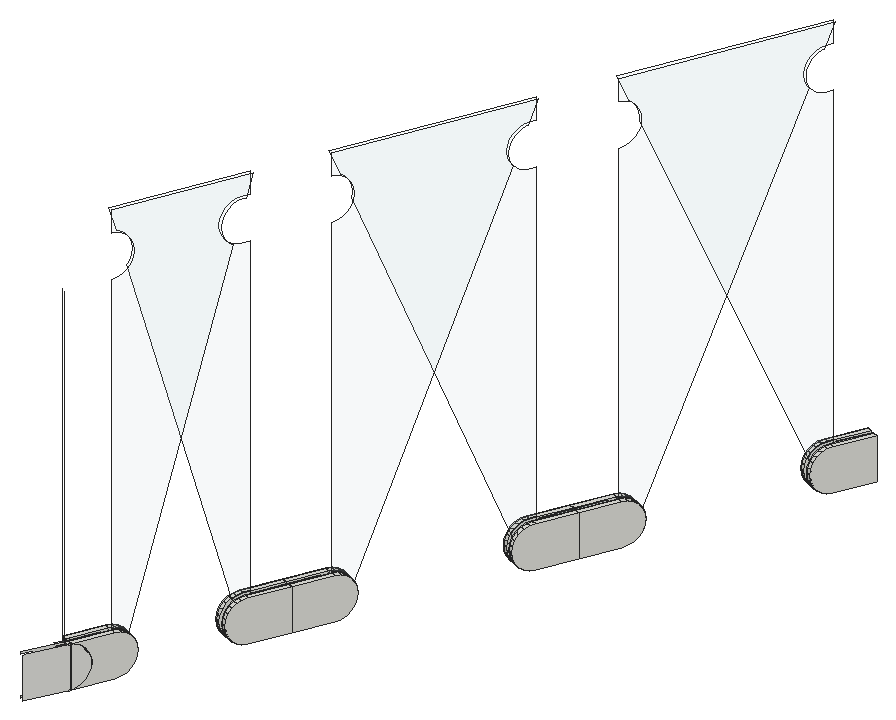
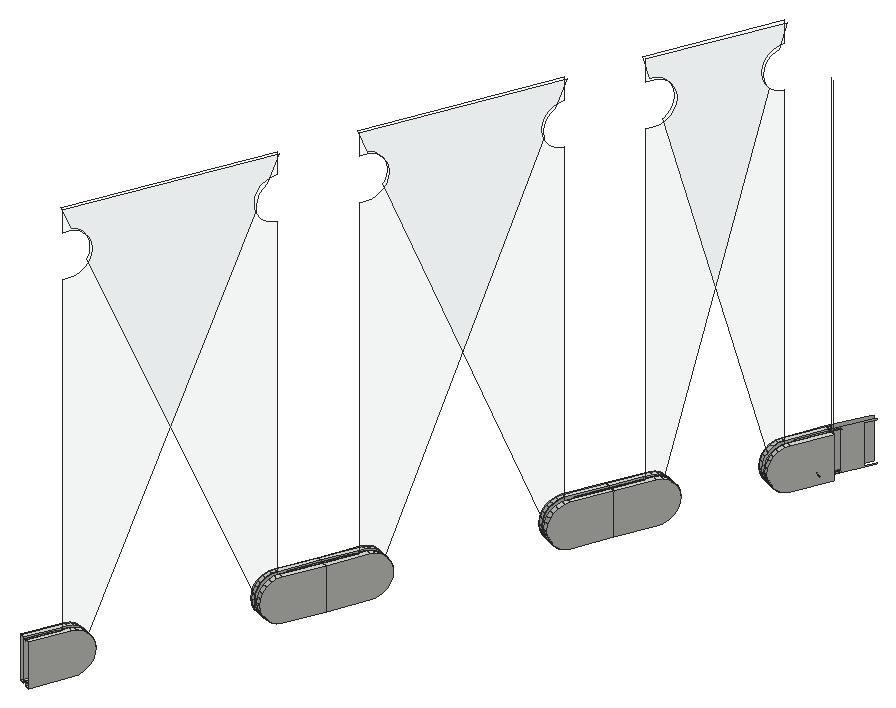
# SketchUp Ruby script. Lengths in inches.
U = 1.inch
M = Sketchup.active_model
def pt(a) = Geom::Point3d.new(a.map { |v| v * U })
def face(e, loops, mat)
  f = e.add_face(loops[0].map { |a| pt(a) })
  loops[1..].each { |l| e.add_face(l.map { |a| pt(a) }).erase! }
  f.material = f.back_material = mat if mat
  f
end
# faces: each face lists its corners as indices into pts; further lists are holes
def faces(e, pts, list, mat = nil) = list.each { |f| face(e, (f[0].is_a?(Array) ? f : [f]).map { |l| l.map { |i| pts[i] } }, mat) }
# xy, xz, yz: faces in a plane at the given z, y or x. An outline is a flat list of corners, or four numbers for a rectangle; further outlines are holes
def ring(l) = l.size == 4 ? [[l[0], l[1]], [l[2], l[1]], [l[2], l[3]], [l[0], l[3]]] : l.each_slice(2).to_a
def flat(e, list, mat, &to3) = list.each { |f| face(e, (f[0].is_a?(Array) ? f : [f]).map { |l| ring(l).map { |u, v| to3.(u, v) } }, mat) }
def xy(e, z, list, mat = nil) = flat(e, list, mat) { |x, y| [x, y, z] }
def xz(e, y, list, mat = nil) = flat(e, list, mat) { |x, z| [x, y, z] }
def yz(e, x, list, mat = nil) = flat(e, list, mat) { |y, z| [x, y, z] }
def lines(e, pts, list) = list.each { |a, b| e.add_line(pt(pts[a]), pt(pts[b])) }
# prism: a flat outline (further loops are holes) pulled along v
def prism(e, loops, v, mat = nil)
  f = face(e, loops, mat); d = Geom::Vector3d.new(v.map { |x| x * U })
  f.pushpull(f.normal.samedirection?(d) ? d.length : -d.length)
end
def box(e, o, s, mat = nil) = prism(e, [[o, [o[0] + s[0], o[1], o[2]], [o[0] + s[0], o[1] + s[1], o[2]], [o[0], o[1] + s[1], o[2]]]], [0, 0, s[2]], mat)
def at(x, y, z, deg = 0) = Geom::Transformation.translation(pt([x, y, z])) * Geom::Transformation.rotation(ORIGIN, Z_AXIS, deg.degrees)
def axes(o, x, y, z) = Geom::Transformation.new([*x, 0, *y, 0, *z, 0, *pt(o).to_a, 1])
def part(name) = M.definitions.add(name)
# library, detail: a bought-in or finely detailed component or shape, given as its bounding box
def library(name, o, s) = part(name).tap { |d| box(d.entities, o, s) }
def detail(e, o, s) = box(e.add_group.entities, o, s)
def put(e, d, t, mat = nil) = e.add_instance(d, t).tap { |i| i.material = mat if mat }
def group(e, t, mat = nil) = e.add_group.tap { |g| g.transformation = t; g.material = mat if mat }.entities
root = M.entities
M.materials.add("Glass_Safety_01").color = [204, 235, 244]
M.materials["Glass_Safety_01"].alpha = 0.1
xy(root,333,[[844.286,537.43,844.039,537.551,844.044,537.562,844.108,537.692,844.355,537.571],[844.362,537.586,844.11,537.696,844.896,539.501,845.148,539.391],[843.931,537.779,843.684,537.9,844.463,539.689,844.715,539.579],[847.571,544.953,847.318,545.063,847.473,545.418,848.104,546.868,848.357,546.758],[847.138,545.142,846.885,545.252,847.671,547.057,847.924,546.947,847.293,545.497,847.167,545.208],
  [848.357,546.758,848.104,546.868,848.89,548.673,849.143,548.563],[847.924,546.947,847.671,547.057,848.457,548.861,848.71,548.751],[852.79,556.936,852.537,557.046,852.656,557.318,853.323,558.851,853.576,558.741],[852.357,557.125,852.104,557.235,852.89,559.04,853.143,558.93,852.475,557.397],[853.576,558.741,853.323,558.851,854.109,560.656,854.362,560.546],
  [853.143,558.93,852.89,559.04,853.676,560.845,853.929,560.735],[858.192,569.34,857.939,569.45,858.054,569.713,858.726,571.255,858.978,571.145],[857.759,569.529,857.506,569.639,858.292,571.443,858.545,571.333,857.873,569.791]])
xy(root,333.078,[[843.866,537.198,843.689,537.285,843.862,537.638,843.867,537.648,843.929,537.775,844.019,537.735,844.108,537.692,844.044,537.562,844.039,537.552],[844.11,537.696,844.019,537.735,843.931,537.779,844.558,539.218,844.738,539.14],[844.019,537.735,843.929,537.775,843.931,537.779],[847.476,545.424,847.295,545.503,847.924,546.947,848.104,546.868],[848.104,546.868,847.924,546.947,848.553,548.39,848.733,548.312],
  [852.695,557.407,852.514,557.486,853.143,558.93,853.323,558.851],[853.323,558.851,853.143,558.93,853.772,560.374,853.952,560.295],[858.097,569.811,857.916,569.89,858.545,571.333,858.726,571.255]],"Glass_Safety_01")
xy(root,335.047,[[843.866,537.198,844.039,537.551,844.04,537.553,844.044,537.562,844.108,537.692,844.019,537.735,843.929,537.775,843.867,537.648,843.867,537.647,843.862,537.638,843.689,537.285],[844.11,537.696,844.738,539.14,844.558,539.218,843.931,537.779,844.019,537.735],[844.019,537.735,843.931,537.779,843.929,537.775],[847.476,545.424,848.104,546.868,847.924,546.947,847.295,545.503],[848.104,546.868,848.733,548.312,848.553,548.39,847.924,546.947],
  [852.695,557.407,853.323,558.851,853.143,558.93,852.514,557.486],[853.323,558.851,853.952,560.295,853.772,560.374,853.143,558.93],[858.097,569.811,858.726,571.255,858.545,571.333,857.916,569.89]],"Glass_Safety_01")
xy(root,335.126,[[844.362,537.586,845.148,539.391,844.896,539.501,844.11,537.696],[843.931,537.779,844.715,539.579,844.463,539.689,843.684,537.9],[847.571,544.953,848.357,546.758,848.104,546.868,847.473,545.418,847.318,545.063],[847.138,545.142,847.293,545.497,847.924,546.947,847.671,547.057,846.885,545.252],[848.357,546.758,849.143,548.563,848.89,548.673,848.104,546.868],
  [847.924,546.947,848.71,548.751,848.457,548.861,847.671,547.057],[852.79,556.936,853.576,558.741,853.323,558.851,852.656,557.318,852.537,557.046],[852.357,557.125,852.475,557.397,853.143,558.93,852.89,559.04,852.104,557.235],[853.576,558.741,854.362,560.546,854.109,560.656,853.323,558.851],[853.143,558.93,853.929,560.735,853.676,560.845,852.89,559.04],
  [858.192,569.34,858.978,571.145,858.726,571.255,858.054,569.713,857.939,569.45],[857.759,569.529,857.873,569.791,858.545,571.333,858.292,571.443,857.506,569.639]])
yz(root,843.867,[[537.648,333.078,537.647,335.047,537.648,335.047]],"Glass_Safety_01")
p = [[843.42,535.662,335.105],[843.42,535.662,333.02],[843.489,535.803,333],[844.286,537.43,333],[844.355,537.571,333.02],[844.355,537.571,335.105],
  [844.286,537.43,335.126],[843.489,535.803,335.126],[843.173,535.784,335.047],[843.173,535.784,335.105],[843.242,535.924,335.126],[844.039,537.551,335.126],
  [844.04,537.553,335.125],[844.044,537.562,335.124],[844.108,537.692,335.105],[844.108,537.692,335.047],[844.044,537.562,335.047],[844.044,537.562,333.078],
  [844.108,537.692,333.078],[844.11,537.696,335.104],[844.16,537.799,335.089],[844.273,538.029,334.983],[844.37,538.226,334.814],[844.444,538.378,334.594],
  [844.491,538.474,334.338],[844.507,538.506,334.0625],[844.491,538.474,333.787],[844.444,538.378,333.531],[844.37,538.226,333.311],[844.273,538.029,333.142],
  [844.16,537.799,333.036],[844.11,537.696,333.021],[844.108,537.692,333.02],[844.044,537.562,333.001],[844.039,537.551,333],[843.242,535.924,333],
  [843.173,535.784,333.02],[843.173,535.784,333.078],[843.415,536.278,333.078],[843.415,536.278,335.047],[844.04,537.553,335.047],[844.039,537.551,335.047],
  [843.866,537.198,335.047],[843.866,537.198,333.078],[844.039,537.552,333.078],[844.407,537.677,333.036],[844.362,537.586,333.022],[844.355,537.571,333],
  [843.867,537.648,333.001],[843.867,537.648,333],[843.862,537.638,333],[843.862,537.638,333.078],[843.867,537.648,333.078],[844.044,537.562,333],
  [844.108,537.692,333],[844.108,537.692,335.126],[844.355,537.571,335.126],[844.11,537.696,333],[844.362,537.586,333],[844.362,537.586,335.103],
  [844.362,537.586,335.126],[844.11,537.696,335.126],[844.11,537.696,335.047],[844.11,537.696,333.078],[844.407,537.677,335.089],[844.52,537.908,333.142],
  [844.617,538.105,333.311],[844.691,538.257,333.531],[844.738,538.352,333.787],[844.754,538.385,334.0625],[844.738,538.352,334.338],[844.691,538.257,334.594],
  [844.617,538.105,334.814],[844.52,537.908,334.983],[845.148,539.391,335.126],[845.148,539.391,333],[845.258,539.643,333.036],[845.361,539.878,333.142],
  [845.448,540.08,333.311],[845.516,540.235,333.531],[845.558,540.332,333.787],[845.573,540.365,334.0625],[845.558,540.332,334.338],[845.516,540.235,334.594],
  [845.448,540.08,334.814],[845.361,539.878,334.983],[845.258,539.643,335.089],[844.896,539.501,335.126],[845.006,539.753,335.089],[845.108,539.988,334.983],
  [845.196,540.19,334.814],[845.219,540.244,334.737],[845.263,540.345,334.594],[845.306,540.442,334.338],[845.32,540.475,334.0625],[845.306,540.442,333.787],
  [845.263,540.345,333.531],[845.196,540.19,333.311],[845.108,539.988,333.142],[845.028,539.805,333.059],[845.006,539.753,333.036],[844.896,539.501,333],
  [843.931,537.779,333],[843.931,537.779,333.02],[843.929,537.775,333.02],[843.929,537.775,333],[843.929,537.775,333.078],[843.931,537.779,333.078],
  [843.931,537.779,335.047],[843.931,537.779,335.105],[843.929,537.775,335.106],[843.929,537.775,335.047],[843.983,537.885,335.089],[843.983,537.885,333.036],
  [844.096,538.115,333.142],[844.193,538.313,333.311],[844.267,538.465,333.531],[844.314,538.56,333.787],[844.33,538.593,334.0625],[844.314,538.56,334.338],
  [844.267,538.465,334.594],[844.193,538.313,334.814],[844.096,538.115,334.983],[843.931,537.779,335.126],[843.929,537.775,335.126],[844.715,539.579,333],
  [844.825,539.832,333.036],[844.927,540.067,333.142],[845.015,540.268,333.311],[845.083,540.423,333.531],[845.125,540.521,333.787],[845.14,540.554,334.0625],
  [845.125,540.521,334.338],[845.083,540.423,334.594],[845.015,540.268,334.814],[844.927,540.067,334.983],[844.825,539.832,335.089],[844.715,539.579,335.126],
  [843.736,538.006,333.036],[843.849,538.237,333.142],[843.684,537.9,333.02],[843.684,537.9,335.105],[843.736,538.006,335.089],[843.849,538.237,334.983],
  [843.945,538.434,334.814],[844.02,538.586,334.594],[844.066,538.681,334.338],[844.082,538.714,334.0625],[844.066,538.681,333.787],[844.02,538.586,333.531],
  [843.945,538.434,333.311],[843.677,537.885,335.126],[843.68,537.892,335.126],[843.684,537.9,335.126],[844.463,539.689,335.126],[844.572,539.942,335.089],
  [844.675,540.177,334.983],[844.763,540.379,334.814],[844.83,540.533,334.594],[844.873,540.631,334.338],[844.887,540.664,334.0625],[844.873,540.631,333.787],
  [844.83,540.533,333.531],[844.763,540.379,333.311],[844.675,540.177,333.142],[844.572,539.942,333.036],[844.463,539.689,333],[843.684,537.9,333],
  [843.68,537.892,333],[843.677,537.885,333],[843.676,537.885,333.018],[843.676,537.885,335.107],[848.357,546.758,335.126],[847.571,544.953,335.126],
  [847.461,544.701,335.089],[847.359,544.466,334.983],[847.271,544.264,334.814],[847.203,544.109,334.594],[847.161,544.012,334.338],[847.147,543.979,334.0625],
  [847.161,544.012,333.787],[847.203,544.109,333.531],[847.271,544.264,333.311],[847.359,544.466,333.142],[847.461,544.701,333.036],[847.571,544.953,333],
  [848.357,546.758,333],[847.318,545.063,335.126],[847.473,545.418,335.126],[847.473,545.418,333],[847.318,545.063,333],[847.208,544.811,333.036],
  [847.106,544.576,333.142],[847.018,544.374,333.311],[846.951,544.219,333.531],[846.908,544.122,333.787],[846.894,544.089,334.0625],[846.908,544.122,334.338],
  [846.951,544.219,334.594],[847.018,544.374,334.814],[847.106,544.576,334.983],[847.208,544.811,335.089],[846.939,544.686,334.997],[846.926,544.655,334.983],
  [846.838,544.453,334.814],[846.77,544.298,334.594],[846.728,544.2,334.338],[846.713,544.167,334.0625],[846.728,544.2,333.787],[846.77,544.298,333.531],
  [846.838,544.453,333.311],[846.926,544.655,333.142],[847.028,544.89,333.036],[847.138,545.142,333],[847.167,545.208,333],[846.885,545.252,335.126],
  [847.671,547.057,335.126],[847.671,547.057,333],[846.885,545.252,333],[846.775,545,333.036],[846.673,544.765,333.142],[846.585,544.563,333.311],
  [846.518,544.408,333.531],[846.475,544.311,333.787],[846.461,544.277,334.0625],[846.475,544.311,334.338],[846.518,544.408,334.594],[846.585,544.563,334.814],
  [846.673,544.765,334.983],[846.775,545,335.089],[847.293,545.497,333],[847.293,545.497,335.126],[847.138,545.142,335.126],[847.028,544.89,335.089],
  [848.104,546.868,333],[848.104,546.868,335.126],[848.104,546.868,335.047],[847.476,545.424,335.047],[847.476,545.424,333.078],[848.104,546.868,333.078],
  [847.924,546.947,335.126],[847.924,546.947,333],[847.924,546.947,333.078],[847.295,545.503,333.078],[847.295,545.503,335.047],[847.924,546.947,335.047],
  [849.143,548.563,335.126],[849.143,548.563,333],[849.253,548.815,333.036],[849.355,549.05,333.142],[849.443,549.252,333.311],[849.511,549.407,333.531],
  [849.553,549.504,333.787],[849.567,549.537,334.0625],[849.553,549.504,334.338],[849.511,549.407,334.594],[849.443,549.252,334.814],[849.355,549.05,334.983],
  [849.253,548.815,335.089],[848.71,548.751,333],[848.71,548.751,335.126],[848.553,548.39,335.047],[848.553,548.39,333.078],[848.89,548.673,335.126],
  [848.89,548.673,333],[848.733,548.312,333.078],[848.733,548.312,335.047],[848.457,548.861,335.126],[848.567,549.114,335.089],[848.669,549.349,334.983],
  [848.757,549.551,334.814],[848.825,549.705,334.594],[848.867,549.803,334.338],[848.882,549.836,334.0625],[848.867,549.803,333.787],[848.825,549.705,333.531],
  [848.757,549.551,333.311],[848.669,549.349,333.142],[848.567,549.114,333.036],[848.457,548.861,333],[849,548.925,333.036],[849.299,549.61,334.349],
  [849.097,549.146,333.136],[849,548.925,335.089],[849.103,549.16,334.983],[849.191,549.362,334.814],[849.258,549.517,334.594],[848.82,549.004,333.036],
  [848.82,549.004,335.089],[848.922,549.239,334.983],[849.01,549.44,334.814],[849.077,549.595,334.594],[849.12,549.693,334.338],[849.134,549.726,334.0625],
  [849.12,549.693,333.787],[849.077,549.595,333.531],[849.01,549.44,333.311],[848.922,549.239,333.142],[849.103,549.16,333.142],[853.576,558.741,335.126],
  [852.79,556.936,335.126],[852.68,556.684,335.089],[852.578,556.449,334.983],[852.49,556.247,334.814],[852.422,556.092,334.594],[852.38,555.995,334.338],
  [852.366,555.962,334.0625],[852.38,555.995,333.787],[852.422,556.092,333.531],[852.49,556.247,333.311],[852.578,556.449,333.142],[852.68,556.684,333.036],
  [852.79,556.936,333],[853.576,558.741,333],[852.537,557.046,335.126],[852.656,557.318,335.126],[852.656,557.318,333],[852.537,557.046,333],
  [852.428,556.794,333.036],[852.325,556.559,333.142],[852.237,556.357,333.311],[852.17,556.202,333.531],[852.127,556.105,333.787],[852.113,556.072,334.0625],
  [852.127,556.105,334.338],[852.17,556.202,334.594],[852.237,556.357,334.814],[852.325,556.559,334.983],[852.428,556.794,335.089],[852.013,556.336,334.672],
  [851.989,556.281,334.594],[851.947,556.184,334.338],[851.932,556.151,334.0625],[851.947,556.184,333.787],[851.989,556.281,333.531],[852.057,556.436,333.311],
  [852.145,556.638,333.142],[852.247,556.873,333.036],[852.288,556.967,333.022],[852.104,557.235,335.126],[852.89,559.04,335.126],[852.89,559.04,333],
  [852.104,557.235,333],[851.994,556.983,333.036],[851.892,556.748,333.142],[851.804,556.546,333.311],[851.737,556.391,333.531],[851.694,556.294,333.787],
  [851.68,556.261,334.0625],[851.694,556.294,334.338],[851.737,556.391,334.594],[851.804,556.546,334.814],[851.892,556.748,334.983],[851.994,556.983,335.089],
  [852.357,557.125,333],[852.475,557.397,333],[852.475,557.397,335.126],[852.357,557.125,335.126],[852.247,556.873,335.089],[852.145,556.638,334.983],
  [852.057,556.436,334.814],[853.323,558.851,333],[853.323,558.851,335.126],[853.323,558.851,335.047],[852.695,557.407,335.047],[852.695,557.407,333.078],
  [853.323,558.851,333.078],[853.143,558.93,335.126],[853.143,558.93,333],[853.143,558.93,333.078],[852.514,557.486,333.078],[852.514,557.486,335.047],
  [853.143,558.93,335.047],[854.362,560.546,335.126],[854.362,560.546,333],[854.472,560.798,333.036],[854.574,561.033,333.142],[854.662,561.235,333.311],
  [854.73,561.39,333.531],[854.772,561.487,333.787],[854.787,561.521,334.0625],[854.772,561.487,334.338],[854.73,561.39,334.594],[854.662,561.235,334.814],
  [854.574,561.033,334.983],[854.472,560.798,335.089],[853.929,560.735,333],[853.929,560.735,335.126],[853.772,560.374,335.047],[853.772,560.374,333.078],
  [854.109,560.656,335.126],[854.109,560.656,333],[853.952,560.295,333.078],[853.952,560.295,335.047],[853.676,560.845,335.126],[853.786,561.097,335.089],
  [853.889,561.332,334.983],[853.976,561.534,334.814],[854.044,561.689,334.594],[854.086,561.786,334.338],[854.101,561.819,334.0625],[854.086,561.786,333.787],
  [854.044,561.689,333.531],[853.976,561.534,333.311],[853.889,561.332,333.142],[853.786,561.097,333.036],[853.676,560.845,333],[854.219,560.908,333.036],
  [854.039,560.987,333.036],[854.039,560.987,335.089],[854.141,561.222,334.983],[854.229,561.424,334.814],[854.297,561.579,334.594],[854.339,561.676,334.338],
  [854.353,561.709,334.0625],[854.339,561.676,333.787],[854.297,561.579,333.531],[854.229,561.424,333.311],[854.141,561.222,333.142],[854.523,561.606,334.269],
  [854.329,561.16,333.156],[854.322,561.143,333.142],[854.219,560.908,335.089],[854.322,561.143,334.983],[854.41,561.345,334.814],[854.477,561.5,334.594],
  [854.519,561.597,334.338],[858.978,571.145,335.126],[858.192,569.34,335.126],[858.082,569.088,335.089],[857.98,568.853,334.983],[857.892,568.651,334.814],
  [857.825,568.496,334.594],[857.782,568.399,334.338],[857.768,568.365,334.0625],[857.782,568.399,333.787],[857.825,568.496,333.531],[857.892,568.651,333.311],
  [857.98,568.853,333.142],[858.082,569.088,333.036],[858.192,569.34,333],[858.978,571.145,333],[857.939,569.45,335.126],[858.054,569.713,335.126],
  [858.054,569.713,333],[857.939,569.45,333],[857.83,569.198,333.036],[857.727,568.963,333.142],[857.639,568.761,333.311],[857.572,568.606,333.531],
  [857.53,568.509,333.787],[857.515,568.475,334.0625],[857.53,568.509,334.338],[857.572,568.606,334.594],[857.639,568.761,334.814],[857.727,568.963,334.983],
  [857.83,569.198,335.089],[857.399,568.702,334.618],[857.391,568.685,334.594],[857.349,568.587,334.338],[857.335,568.554,334.0625],[857.349,568.587,333.787],
  [857.391,568.685,333.531],[857.459,568.839,333.311],[857.547,569.041,333.142],[857.649,569.276,333.036],[857.676,569.339,333.027],[857.506,569.639,335.126],
  [858.292,571.443,335.126],[858.292,571.443,333],[857.506,569.639,333],[857.396,569.386,333.036],[857.294,569.151,333.142],[857.206,568.95,333.311],
  [857.139,568.795,333.531],[857.096,568.697,333.787],[857.082,568.664,334.0625],[857.096,568.697,334.338],[857.139,568.795,334.594],[857.206,568.95,334.814],
  [857.294,569.151,334.983],[857.396,569.386,335.089],[857.759,569.529,333],[857.873,569.791,333],[857.873,569.791,335.126],[857.759,569.529,335.126],
  [857.649,569.276,335.089],[857.547,569.041,334.983],[857.459,568.839,334.814],[858.726,571.255,333],[858.726,571.255,335.126],[858.726,571.255,335.047],
  [858.097,569.811,335.047],[858.097,569.811,333.078],[858.726,571.255,333.078],[858.545,571.333,335.126],[858.545,571.333,333],[858.545,571.333,333.078],
  [857.916,569.89,333.078],[857.916,569.89,335.047],[858.545,571.333,335.047],[843.867,537.648,335.047],[844.019,537.735,333.078],[844.019,537.735,335.047],
  [844.738,539.14,333.078],[844.738,539.14,335.047],[843.93,537.777,335.047],[843.93,537.777,333.078],[844.558,539.218,333.078],[844.558,539.218,335.047],
  [849.191,549.362,333.311],[849.258,549.517,333.531],[849.3,549.614,333.787],[849.315,549.647,334.0625],[849.3,549.614,334.338],[854.41,561.345,333.311],
  [854.477,561.5,333.531],[854.519,561.597,333.787],[854.534,561.631,334.0625],[848.89,548.673,351.283],[852.194,556.257,351.736],[852.17,556.202,351.815],
  [852.127,556.105,352.071],[852.113,556.072,352.346],[852.127,556.105,352.621],[852.17,556.202,352.877],[852.237,556.357,353.098],[852.325,556.559,353.267],
  [852.428,556.794,353.373],[852.468,556.888,353.386],[852.656,557.318,354.511],[848.89,548.673,354.511],[848.89,548.673,353.409],[849,548.925,353.373],
  [849.103,549.16,353.267],[849.191,549.362,353.098],[849.258,549.517,352.877],[849.3,549.614,352.621],[849.315,549.647,352.346],[849.3,549.614,352.071],
  [849.258,549.517,351.815],[849.191,549.362,351.594],[849.103,549.16,351.425],[849,548.925,351.319],[854.109,560.656,351.283],[857.579,568.623,351.79],
  [857.572,568.606,351.815],[857.53,568.509,352.071],[857.515,568.475,352.346],[857.53,568.509,352.621],[857.572,568.606,352.877],[857.639,568.761,353.098],
  [857.727,568.963,353.267],[857.83,569.198,353.373],[857.857,569.26,353.382],[858.054,569.713,354.511],[854.109,560.656,354.511],[854.109,560.656,353.409],
  [854.219,560.908,353.373],[854.322,561.143,353.267],[854.41,561.345,353.098],[854.477,561.5,352.877],[854.519,561.597,352.621],[854.534,561.631,352.346],
  [854.519,561.597,352.071],[854.477,561.5,351.815],[854.41,561.345,351.594],[854.322,561.143,351.425],[854.219,560.908,351.319],[854.343,561.684,352.14],
  [854.353,561.709,352.346],[854.339,561.676,352.621],[854.297,561.579,352.877],[854.229,561.424,353.098],[854.149,561.239,353.252],[853.929,560.735,354.511],
  [857.873,569.791,354.511],[857.873,569.791,353.409],[857.759,569.529,353.409],[857.649,569.276,353.373],[857.547,569.041,353.267],[857.459,568.839,353.098],
  [857.391,568.685,352.877],[857.349,568.587,352.621],[857.335,568.554,352.346],[857.349,568.587,352.071],[857.391,568.685,351.815],[857.459,568.839,351.594],
  [857.547,569.041,351.425],[857.649,569.276,351.319],[857.759,569.529,351.283],[857.873,569.791,351.283],[847.12,544.607,351.411],[847.106,544.576,351.425],
  [847.018,544.374,351.594],[846.951,544.219,351.815],[846.908,544.122,352.071],[846.894,544.089,352.346],[846.908,544.122,352.621],[846.951,544.219,352.877],
  [847.018,544.374,353.098],[847.106,544.576,353.267],[847.208,544.811,353.373],[847.318,545.063,353.409],[847.347,545.13,353.409],[847.473,545.418,354.511],
  [844.896,539.501,354.511],[844.896,539.501,353.409],[845.006,539.753,353.373],[845.108,539.988,353.267],[845.196,540.19,353.098],[845.263,540.345,352.877],
  [845.306,540.442,352.621],[845.32,540.475,352.346],[845.306,540.442,352.071],[845.263,540.345,351.815],[845.196,540.19,351.594],[845.108,539.988,351.425],
  [845.006,539.753,351.319],[844.896,539.501,351.283],[849.118,549.689,352.06],[849.12,549.693,352.071],[849.134,549.726,352.346],[849.12,549.693,352.621],
  [849.077,549.595,352.877],[849.01,549.44,353.098],[848.922,549.239,353.267],[848.916,549.225,353.273],[848.71,548.751,354.511],[852.475,557.397,354.511],
  [852.475,557.397,353.409],[852.357,557.125,353.409],[852.247,556.873,353.373],[852.145,556.638,353.267],[852.057,556.436,353.098],[851.989,556.281,352.877],
  [851.947,556.184,352.621],[851.932,556.151,352.346],[851.947,556.184,352.071],[851.989,556.281,351.815],[852.057,556.436,351.594],[852.145,556.638,351.425],
  [852.247,556.873,351.319],[852.357,557.125,351.283],[852.475,557.397,351.283],[843.867,537.647,335.126],[843.863,537.64,351.283],[843.867,537.648,351.283],
  [843.867,537.648,335.126],[843.867,537.648,335.124],[843.867,537.647,335.047],[843.867,537.647,335.124],[845.039,540.323,351.671],[845.083,540.423,351.815],
  [845.125,540.521,352.071],[845.14,540.554,352.346],[845.125,540.521,352.621],[845.083,540.423,352.877],[845.015,540.268,353.098],[844.927,540.067,353.267],
  [844.848,539.883,353.349],[844.715,539.579,354.511],[847.293,545.497,354.511],[847.293,545.497,353.409],[847.138,545.142,353.409],[847.028,544.89,353.373],
  [846.926,544.655,353.267],[846.838,544.453,353.098],[846.77,544.298,352.877],[846.728,544.2,352.621],[846.713,544.167,352.346],[846.728,544.2,352.071],
  [846.77,544.298,351.815],[846.838,544.453,351.594],[846.926,544.655,351.425],[847.028,544.89,351.319],[847.138,545.142,351.283],[847.293,545.497,351.283],
  [844.044,537.562,335.126],[844.039,537.551,351.283],[844.043,537.56,351.283],[844.044,537.562,351.283]]
faces(root,p,[[0,1,2,3,4,5,6,7],[[8,9,10,11,12,13,14,15,16,17,18,15,14,19,20,21,22,23,24,25,26,27,28,29,30,31,32,33,34,35,36,37,38,39],[40,41,42,43,44]],[31,30,45,46,4,3,34,33,32],[47,4,3],[54,53,33,32],[54,32,18,15,14,55,56,5,4,47],[31,57,58,46,59,60,61,19,62,63],[4,46,59,5],
  [64,59,46,45,65,66,67,68,69,70,71,72,73],[74,60,59,46,58,75,76,77,78,79,80,81,82,83,84,85,86],[61,87,88,89,90,91,92,93,94,95,96,97,98,99,100,101,57,31,63,62,19],[30,29,65,45],[102,103,104,105],[106,104,103,107,108,109,110,111],[112,109,108,107,103,113,114,115,116,117,118,119,120,121,122],[123,124,110,111,106,104,105,102,125,126,127,128,129,130,131,132,133,134,135,136,137],
  [114,113,138,139],[138,140,141,142,143,144,145,146,147,148,149,150,139],[151,152,153,154,155,156,157,158,159,160,161,162,163,164,165,166,167,168,169,170,171],[101,100,76,75],[126,125,166,165],[99,98,77,76,100],[127,126,165,164],[172,173,174,175,176,177,178,179,180,181,182,183,184,185,186],
  [187,188,189,190,191,192,193,194,195,196,197,198,199,200,201],[202,203,204,205,206,207,208,209,210,211,212,213,214],[215,216,217,218,219,220,221,222,223,224,225,226,227,228,229],[192,191,184,183],[212,211,220,219],[191,190,185,184],[213,212,219,218],[234,189,188,235,236,237,238,239],
  [240,231,230,241,242,243,244,245],[234,239,236,235,172,186],[246,172,186,247,248,249,250,251,252,253,254,255,256,257,258],[242,241,217,216,240,245],[241,259,260,240,245,261,262,242],[235,263,264,234,239,265,266,236],[216,267,268,269,270,271,272,273,274,275,276,277,278,279,217],[264,280,248,247],
  [287,259,279,278],[282,298,249,248,280],[297,287,278,277],[299,300,301,302,303,304,305,306,307,308,309,310,311,312,313],[314,315,316,317,318,319,320,321,322,323,324,325,326,327,328],[329,330,331,332,333,334,335,336,337,338],[339,340,341,342,343,344,345,346,347,348,349,350,351,352,353],[319,318,311,310],
  [337,336,344,343],[318,317,312,311],[338,337,343,342,354],[361,316,315,362,363,364,365,366],[367,356,355,368,369,370,371,372],[361,366,363,362,299,313],[373,299,313,374,375,376,377,378,379,380,381,382,383,384,385],[369,368,341,340,367,372],
  [368,386,387,367,372,388,389,369],[362,390,391,361,366,392,393,363],[340,394,395,396,397,398,399,400,401,402,403,404,405,406,341],[391,407,375,374],[408,386,406,405],[407,421,376,375],[418,408,405,404],[427,428,429,430,431,432,433,434,435,436,437,438,439,440,441],
  [442,443,444,445,446,447,448,449,450,451,452,453,454,455,456],[457,458,459,460,461,462,463,464,465,466],[467,468,469,470,471,472,473,474,475,476,477,478,479,480,481],[447,446,439,438],[465,464,472,471],[446,445,440,439],[466,465,471,470,482],[489,444,443,490,491,492,493,494],
  [495,484,483,496,497,498,499,500],[29,28,66,65],[115,114,139,150],[98,97,78,77],[128,127,164,163],[193,192,183,182],[211,210,221,220],[298,510,250,249],
  [296,297,277,276],[320,319,310,309],[336,335,345,344],[420,515,377,376,421],[417,418,404,403],[448,447,438,437],[464,463,473,472],[28,27,67,66],
  [116,115,150,149],[97,96,79,78],[129,128,163,162],[194,193,182,181],[210,209,222,221],[510,511,251,250],[295,296,276,275],[321,320,309,308],
  [335,334,346,345],[515,516,378,377],[416,417,403,402],[449,448,437,436],[463,462,474,473],[27,26,68,67],[117,116,149,148],[96,95,80,79],
  [130,129,162,161],[195,194,181,180],[209,208,223,222],[511,512,252,251],[294,295,275,274],[322,321,308,307],[334,333,347,346],[516,517,379,378],
  [415,416,402,401],[450,449,436,435],[462,461,475,474],[26,25,69,68],[118,117,148,147],[95,94,81,80],[131,130,161,160],[196,195,180,179],
  [208,207,224,223],[512,513,253,252],[293,294,274,273],[323,322,307,306],[333,332,348,347],[517,518,380,379],[414,415,401,400],[451,450,435,434],
  [461,460,476,475],[25,24,70,69],[119,118,147,146],[94,93,82,81],[132,131,160,159],[197,196,179,178],[207,206,225,224],[513,514,254,253],
  [292,293,273,272],[324,323,306,305],[332,331,349,348],[419,426,381,380,518],[413,414,400,399],[452,451,434,433],[460,459,477,476],[24,23,71,70],
  [120,119,146,145],[93,92,83,82],[133,132,159,158],[198,197,178,177],[206,205,226,225],[281,286,255,254,514],[291,292,272,271],[325,324,305,304],
  [331,330,350,349],[426,425,382,381],[412,413,399,398],[453,452,433,432],[459,458,478,477],[23,22,72,71],[121,120,145,144],[91,90,84,83,92],
  [134,133,158,157],[199,198,177,176],[205,204,227,226],[286,285,256,255],[290,291,271,270],[326,325,304,303],[329,360,351,350,330],[425,424,383,382],
  [411,412,398,397],[454,453,432,431],[457,488,479,478,458],[22,21,73,72],[122,121,144,143],[90,89,85,84],[135,134,157,156],[200,199,176,175],
  [204,203,228,227],[285,284,257,256],[289,290,270,269],[327,326,303,302],[360,359,352,351],[424,423,384,383],[410,411,397,396],[455,454,431,430],
  [488,487,480,479],[21,20,64,73],[112,122,143,142],[89,88,86,85],[136,135,156,155],[201,200,175,174],[202,233,229,228,203],[284,283,258,257],
  [288,289,269,268],[328,327,302,301],[359,358,353,352],[423,422,385,384],[409,410,396,395],[456,455,430,429],[487,486,481,480],[55,678,12,11,6,56],
  [12,11,6,5,59,64,20,19,14,13],[56,6,5],[14,13,678,55],[124,110,109,123],[88,87,74,86],[137,136,155,154],[187,201,174,173],[233,232,215,229],
  [283,263,246,258],[260,288,268,267],[314,328,301,300],[358,357,339,353],[422,390,373,385],[387,409,395,394],[442,456,429,428],[486,485,467,481]])
faces(root,p,[[48,49,50,51,52],[44,34,53,33,17],[87,101,100,99,91,90,89,88],[125,137,136,135,134,133,132,131,130,129,128,127,126],[202,214,230,231,232,233],[281,282,280,264,263,283,284,285,286],[259,260,288,289,290,291,292,293,294,295,296,297,287],[329,338,354,355,356,357,358,359,360],
  [386,387,409,410,411,412,413,414,415,416,417,418,408],[419,420,421,407,391,390,422,423,424,425,426],[457,466,482,483,484,485,486,487,488],[44,43,42,41],[106,52,501,111],[40,44,41],[17,44,41,40,16],[16,17,44,40],
  [16,15,18,17],[502,503,111,106],[108,503,502,107],[18,502,503,15],[503,502,63,62],[63,504,505,62],[506,108,107,507,106,111],[508,107,108,509],
  [504,508,509,505],[91,99,98,97,96,95,94,93,92],[238,237,244,243],[239,238,237,236],[243,242,245,244],[245,236,239,242],[242,262,261,245],[265,239,236,266],
  [266,265,262,261],[281,282,298,510,511,512,513,514],[365,364,371,370],[366,365,364,363],[370,369,372,371],[372,363,366,369],[369,389,388,372],[392,366,363,393],
  [393,392,389,388],[493,492,499,498],[494,493,492,491],[419,420,515,516,517,518],[519,263,283,284,285,286,281,520,521,522,523,524,525,526,527,528,529,530,531,532,533,534,535,536,537,538,539,540,541,542,543],[544,390,422,423,424,425,426,419,545,546,547,548,549,550,551,552,553,554,555,556,557,558,559,560,561,562,563,564,565,566,567,568],[457,569,570,571,572,573,574,575,576,577,578,579,580,581,582,583,584,585,586,587,588,589,590,591,484,485,486,487,488],[91,592,593,594,595,596,597,598,599,600,601,602,603,604,605,606,607,608,609,610,611,612,613,614,615,616,617,618,619,87,88,89,90],
  [329,620,621,622,623,624,625,626,627,628,629,630,631,632,633,634,635,636,637,638,639,640,641,642,643,644,356,357,358,359,360],[645,646,647,648,649,501,650,651],[40,12,11,41],[13,16,40,12],[202,652,653,654,655,656,657,658,659,660,661,662,663,664,665,666,667,668,669,670,671,672,673,674,675,676,677,231,232,233],[679,11,12,680],[680,12,678,681]],"Glass_Safety_01")
